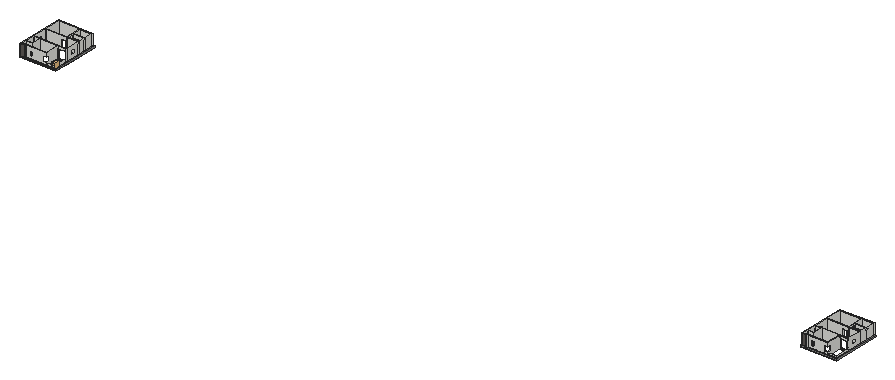
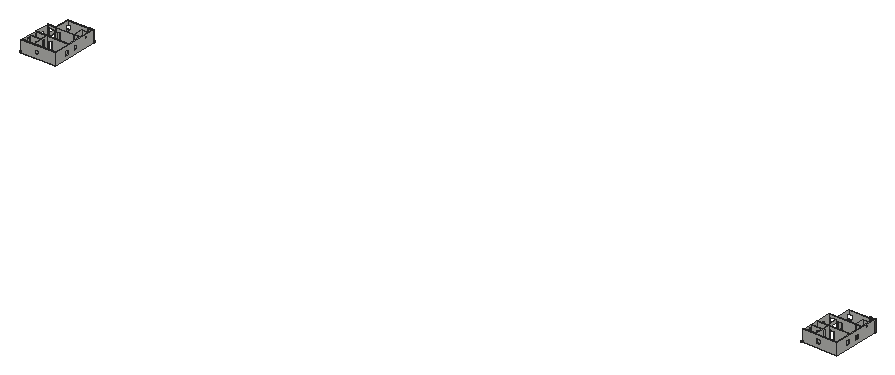
# SketchUp Ruby script. Lengths in inches.
U = 1.inch
M = Sketchup.active_model
def pt(a) = Geom::Point3d.new(a.map { |v| v * U })
def face(e, loops, mat)
  f = e.add_face(loops[0].map { |a| pt(a) })
  loops[1..].each { |l| e.add_face(l.map { |a| pt(a) }).erase! }
  f.material = f.back_material = mat if mat
  f
end
# faces: each face lists its corners as indices into pts; further lists are holes
def faces(e, pts, list, mat = nil) = list.each { |f| face(e, (f[0].is_a?(Array) ? f : [f]).map { |l| l.map { |i| pts[i] } }, mat) }
# xy, xz, yz: faces in a plane at the given z, y or x. An outline is a flat list of corners, or four numbers for a rectangle; further outlines are holes
def ring(l) = l.size == 4 ? [[l[0], l[1]], [l[2], l[1]], [l[2], l[3]], [l[0], l[3]]] : l.each_slice(2).to_a
def flat(e, list, mat, &to3) = list.each { |f| face(e, (f[0].is_a?(Array) ? f : [f]).map { |l| ring(l).map { |u, v| to3.(u, v) } }, mat) }
def xy(e, z, list, mat = nil) = flat(e, list, mat) { |x, y| [x, y, z] }
def xz(e, y, list, mat = nil) = flat(e, list, mat) { |x, z| [x, y, z] }
def yz(e, x, list, mat = nil) = flat(e, list, mat) { |y, z| [x, y, z] }
def lines(e, pts, list) = list.each { |a, b| e.add_line(pt(pts[a]), pt(pts[b])) }
# prism: a flat outline (further loops are holes) pulled along v
def prism(e, loops, v, mat = nil)
  f = face(e, loops, mat); d = Geom::Vector3d.new(v.map { |x| x * U })
  f.pushpull(f.normal.samedirection?(d) ? d.length : -d.length)
end
def box(e, o, s, mat = nil) = prism(e, [[o, [o[0] + s[0], o[1], o[2]], [o[0] + s[0], o[1] + s[1], o[2]], [o[0], o[1] + s[1], o[2]]]], [0, 0, s[2]], mat)
def at(x, y, z, deg = 0) = Geom::Transformation.translation(pt([x, y, z])) * Geom::Transformation.rotation(ORIGIN, Z_AXIS, deg.degrees)
def axes(o, x, y, z) = Geom::Transformation.new([*x, 0, *y, 0, *z, 0, *pt(o).to_a, 1])
def part(name) = M.definitions.add(name)
# library, detail: a bought-in or finely detailed component or shape, given as its bounding box
def library(name, o, s) = part(name).tap { |d| box(d.entities, o, s) }
def detail(e, o, s) = box(e.add_group.entities, o, s)
def put(e, d, t, mat = nil) = e.add_instance(d, t).tap { |i| i.material = mat if mat }
def group(e, t, mat = nil) = e.add_group.tap { |g| g.transformation = t; g.material = mat if mat }.entities
root = M.entities
M.materials.add("Bricks A03 100cm").color = [95, 90, 86]
M.materials.add("Wall Paint Bumpy 01 Gray 100cm").color = [135, 135, 135]
M.materials.add("Wood Amboyan 13.2cm").color = [255, 255, 255]
c1 = part("Vertical board")
xy(c1.entities,0,[[0,0,0.875,8.5625]])
xy(c1.entities,120,[[0,0,0.875,8.5625]])
xz(c1.entities,0,[[0,0,0.875,120]],"Wood Amboyan 13.2cm")
xz(c1.entities,8.5625,[[0,0,0.875,120]])
yz(c1.entities,0,[[0,0,8.5625,120]],"Wood Amboyan 13.2cm")
yz(c1.entities,0.875,[[0,0,8.5625,120]])
c2 = part("Group\#13")
xy(c2.entities,0,[[0,0,45.06,8.5625]])
xy(c2.entities,120.375,[[0,0,45.06,8.5625]])
xz(c2.entities,0,[[0,0,45.06,120.375]],"Bricks A03 100cm")
xz(c2.entities,8.5625,[[0,0,45.06,120.375]])
yz(c2.entities,0,[[0,0,8.5625,120.375]],"Bricks A03 100cm")
yz(c2.entities,45.06,[[0,0,8.5625,120.375]])
c3 = library("Potted Plant 02",[-16.98,-19.78,0],[30.04,38.68,37.52])
xy(root,140.75,[[[420.73,302.125,771.73,779.125],[429.73,311.125,762.73,770.125]],[771.73,302.125,775.4,423.0625],[677.23,311.125,677.23,455.125,672.73,455.125,672.73,459.625,762.73,459.625,762.73,450.625,681.73,450.625,681.73,311.125],[429.73,360.625,452.23,365.125],[485.23,360.625,485.23,365.125,489.73,365.125,489.73,455.125,429.73,455.125,429.73,459.625,633.73,459.625,633.73,455.125,494.23,455.125,494.23,360.625],
  [[8188.44,513.4,8539.44,990.4],[8197.44,522.4,8530.44,981.4]],[8444.94,522.4,8444.94,666.4,8440.44,666.4,8440.44,670.9,8530.44,670.9,8530.44,661.9,8449.44,661.9,8449.44,522.4],[8197.44,571.9,8219.94,576.4],[8252.94,571.9,8252.94,576.4,8257.44,576.4,8257.44,666.4,8197.44,666.4,8197.44,670.9,8401.44,670.9,8401.44,666.4,8261.94,666.4,8261.94,571.9],[429.73,603.625,594.73,608.125],
  [633.73,603.625,633.73,608.125,645.73,608.125,645.73,644.125,650.23,644.125,650.23,608.125,762.73,608.125,762.73,603.625],[645.73,680.125,645.73,770.125,650.23,770.125,650.23,684.625,671.23,684.625,671.23,680.125],[704.23,680.125,762.73,684.625],[8197.44,814.9,8362.44,819.4],[8401.44,814.9,8401.44,819.4,8413.44,819.4,8413.44,855.4,8417.94,855.4,8417.94,819.4,8530.44,819.4,8530.44,814.9],
  [8413.44,891.4,8413.44,981.4,8417.94,981.4,8417.94,895.9,8438.94,895.9,8438.94,891.4],[8471.94,891.4,8530.44,895.9]])
xy(root,140.75,[[420.73,290.125,420.73,293.5625,475.97,293.5625,475.97,302.125,775.4,302.125,775.4,423.0625,786.73,423.0625,786.73,290.125],[771.73,423.0625,786.73,779.125],[8188.44,501.4,8188.44,504.84,8243.6875,504.84,8243.6875,513.4,8539.44,513.4,8539.44,990.4,8554.44,990.4,8554.44,501.4]],"Wall Paint Bumpy 01 Gray 100cm")
xz(root,290.125,[[420.73,140.75,786.73,152.75]],"Wall Paint Bumpy 01 Gray 100cm")
xz(root,293.5625,[[420.73,140.75,475.97,152.75]],"Wall Paint Bumpy 01 Gray 100cm")
xz(root,302.125,[[[420.73,140.75,475.97,140.75,475.97,152.75,681.73,152.75,681.73,176.75,641.23,176.75,641.23,224.75,681.73,224.75,681.73,260.75,420.73,260.75],[512.01,176.75,548.01,224.75]]])
xz(root,302.125,[[475.97,140.75,771.73,152.75]],"Wall Paint Bumpy 01 Gray 100cm")
xz(root,311.125,[[[429.73,140.75,429.73,260.75,677.23,260.75,677.23,224.75,641.23,224.75,641.23,176.75,677.23,176.75,677.23,140.75],[512.01,176.75,548.01,224.75]],[681.73,140.75,762.73,169.375]])
xz(root,360.625,[[429.73,140.75,452.23,140.75,452.23,224.75,485.23,224.75,485.23,140.75,494.23,140.75,494.23,260.75,429.73,260.75]])
xz(root,365.125,[[429.73,140.75,429.73,260.75,489.73,260.75,489.73,140.75,485.23,140.75,485.23,224.75,452.23,224.75,452.23,140.75]])
xz(root,450.625,[[[681.73,140.75,762.73,260.75],[686.23,144.75,758.23,240.75]]])
xz(root,455.125,[[429.73,140.75,489.73,260.75],[494.23,140.75,633.73,140.75,633.73,224.75,672.73,224.75,672.73,140.75,677.23,140.75,677.23,260.75,494.23,260.75]])
xz(root,459.625,[[[429.73,140.75,429.73,260.75,762.73,260.75,762.73,140.75,672.73,140.75,672.73,224.75,633.73,224.75,633.73,140.75],[686.23,144.75,758.23,240.75]]])
xz(root,501.4,[[8188.44,140.75,8554.44,152.75]],"Wall Paint Bumpy 01 Gray 100cm")
xz(root,504.84,[[8188.44,140.75,8243.6875,152.75]],"Wall Paint Bumpy 01 Gray 100cm")
xz(root,513.4,[[[8188.44,140.75,8243.6875,140.75,8243.6875,152.75,8449.44,152.75,8449.44,176.75,8408.94,176.75,8408.94,224.75,8449.44,224.75,8449.44,260.75,8188.44,260.75],[8279.73,176.75,8315.73,224.75]]])
xz(root,513.4,[[8243.6875,140.75,8539.44,152.75]],"Wall Paint Bumpy 01 Gray 100cm")
xz(root,522.4,[[[8197.44,140.75,8197.44,260.75,8444.94,260.75,8444.94,224.75,8408.94,224.75,8408.94,176.75,8444.94,176.75,8444.94,140.75],[8279.73,176.75,8315.73,224.75]],[8449.44,140.75,8530.44,169.375]])
xz(root,571.9,[[8197.44,140.75,8219.94,140.75,8219.94,224.75,8252.94,224.75,8252.94,140.75,8261.94,140.75,8261.94,260.75,8197.44,260.75]])
xz(root,576.4,[[8197.44,140.75,8197.44,260.75,8257.44,260.75,8257.44,140.75,8252.94,140.75,8252.94,224.75,8219.94,224.75,8219.94,140.75]])
xz(root,603.625,[[429.73,140.75,594.73,140.75,594.73,224.75,633.73,224.75,633.73,140.75,762.73,140.75,762.73,260.75,429.73,260.75]])
xz(root,608.125,[[429.73,140.75,429.73,260.75,645.73,260.75,645.73,140.75,633.73,140.75,633.73,224.75,594.73,224.75,594.73,140.75],[650.23,140.75,762.73,260.75]])
xz(root,644.125,[[645.73,140.75,650.23,248.75]])
xz(root,661.9,[[[8449.44,140.75,8530.44,260.75],[8453.94,144.75,8525.94,240.75]]])
xz(root,666.4,[[8197.44,140.75,8257.44,260.75],[8261.94,140.75,8401.44,140.75,8401.44,224.75,8440.44,224.75,8440.44,140.75,8444.94,140.75,8444.94,260.75,8261.94,260.75]])
xz(root,670.9,[[[8197.44,140.75,8197.44,260.75,8530.44,260.75,8530.44,140.75,8440.44,140.75,8440.44,224.75,8401.44,224.75,8401.44,140.75],[8453.94,144.75,8525.94,240.75]]])
xz(root,680.125,[[645.73,140.75,650.23,248.75],[650.23,140.75,671.23,140.75,671.23,224.75,704.23,224.75,704.23,140.75,762.73,140.75,762.73,260.75,650.23,260.75]])
xz(root,684.625,[[650.23,140.75,650.23,260.75,762.73,260.75,762.73,140.75,704.23,140.75,704.23,224.75,671.23,224.75,671.23,140.75]])
xz(root,770.125,[[[429.73,140.75,645.73,260.75],[590.04,176.75,638.04,224.75]],[645.73,140.75,650.23,260.75],[650.23,140.75,762.73,260.75]])
xz(root,779.125,[[[420.73,140.75,771.73,260.75],[590.04,176.75,638.04,224.75]]])
xz(root,779.125,[[771.73,140.75,786.73,152.75]],"Wall Paint Bumpy 01 Gray 100cm")
xz(root,814.9,[[8197.44,140.75,8362.44,140.75,8362.44,224.75,8401.44,224.75,8401.44,140.75,8530.44,140.75,8530.44,260.75,8197.44,260.75]])
xz(root,819.4,[[8197.44,140.75,8197.44,260.75,8413.44,260.75,8413.44,140.75,8401.44,140.75,8401.44,224.75,8362.44,224.75,8362.44,140.75],[8417.94,140.75,8530.44,260.75]])
xz(root,855.4,[[8413.44,140.75,8417.94,248.75]])
xz(root,891.4,[[8413.44,140.75,8417.94,248.75],[8417.94,140.75,8438.94,140.75,8438.94,224.75,8471.94,224.75,8471.94,140.75,8530.44,140.75,8530.44,260.75,8417.94,260.75]])
xz(root,895.9,[[8417.94,140.75,8417.94,260.75,8530.44,260.75,8530.44,140.75,8471.94,140.75,8471.94,224.75,8438.94,224.75,8438.94,140.75]])
xz(root,981.4,[[[8197.44,140.75,8413.44,260.75],[8357.75,176.75,8405.75,224.75]],[8413.44,140.75,8417.94,260.75],[8417.94,140.75,8530.44,260.75]])
xz(root,990.4,[[[8188.44,140.75,8539.44,260.75],[8357.75,176.75,8405.75,224.75]]])
xz(root,990.4,[[8539.44,140.75,8554.44,152.75]],"Wall Paint Bumpy 01 Gray 100cm")
yz(root,420.73,[[[302.125,140.75,779.125,260.75],[618.96,176.75,666.96,224.75],[507.625,176.75,555.625,224.75],[387.69,230.75,411.65,248.75]]])
yz(root,420.73,[[290.125,140.75,293.5625,152.75]],"Wall Paint Bumpy 01 Gray 100cm")
yz(root,429.73,[[311.125,140.75,360.625,260.75],[360.625,140.75,365.125,260.75],[[365.125,140.75,455.125,260.75],[387.69,230.75,411.65,248.75]],[455.125,140.75,459.625,260.75],[[459.625,140.75,603.625,260.75],[507.625,176.75,555.625,224.75]],
  [603.625,140.75,608.125,260.75],[[608.125,140.75,770.125,260.75],[618.96,176.75,666.96,224.75]]])
yz(root,452.23,[[360.625,140.75,365.125,224.75]])
yz(root,475.97,[[293.5625,140.75,302.125,152.75]],"Wall Paint Bumpy 01 Gray 100cm")
yz(root,485.23,[[360.625,140.75,365.125,224.75]])
yz(root,489.73,[[365.125,140.75,455.125,260.75]])
yz(root,494.23,[[360.625,140.75,455.125,260.75]])
yz(root,594.73,[[603.625,140.75,608.125,224.75]])
yz(root,633.73,[[455.125,140.75,459.625,224.75],[603.625,140.75,608.125,224.75]])
yz(root,645.73,[[608.125,140.75,608.125,260.75,770.125,260.75,770.125,140.75,680.125,140.75,680.125,248.75,644.125,248.75,644.125,140.75]])
yz(root,650.23,[[608.125,140.75,644.125,140.75,644.125,248.75,680.125,248.75,680.125,260.75,608.125,260.75],[684.625,140.75,770.125,260.75]])
yz(root,671.23,[[680.125,140.75,684.625,224.75]])
yz(root,672.73,[[455.125,140.75,459.625,224.75]])
yz(root,677.23,[[311.125,140.75,311.125,176.75,335.125,176.75,335.125,224.75,311.125,224.75,311.125,260.75,455.125,260.75,455.125,140.75]])
yz(root,681.73,[[311.125,140.75,450.25,140.75,450.25,259.75,325.25,259.75,325.25,260.75,302.125,260.75,302.125,224.75,335.125,224.75,335.125,176.75,302.125,176.75,302.125,170.375,311.125,170.375],[450.25,140.75,450.625,260.75]])
yz(root,704.23,[[680.125,140.75,684.625,224.75]])
yz(root,762.73,[[311.125,140.75,450.625,169.375],[450.625,140.75,459.625,260.75],[[459.625,140.75,603.625,260.75],[507.625,176.75,555.625,224.75]],[603.625,140.75,608.125,260.75],[608.125,140.75,680.125,260.75],
  [680.125,140.75,684.625,260.75],[[684.625,140.75,770.125,260.75],[691.19,230.75,715.15,248.75]]])
yz(root,771.73,[[302.125,140.75,779.125,152.75]],"Wall Paint Bumpy 01 Gray 100cm")
yz(root,786.73,[[290.125,140.75,779.125,152.75]],"Wall Paint Bumpy 01 Gray 100cm")
yz(root,8188.44,[[[513.4,140.75,990.4,260.75],[830.24,176.75,878.24,224.75],[718.9,176.75,766.9,224.75],[598.97,230.75,622.93,248.75]]])
yz(root,8188.44,[[501.4,140.75,504.84,152.75]],"Wall Paint Bumpy 01 Gray 100cm")
yz(root,8197.44,[[522.4,140.75,571.9,260.75],[571.9,140.75,576.4,260.75],[[576.4,140.75,666.4,260.75],[598.97,230.75,622.93,248.75]],[666.4,140.75,670.9,260.75],[[670.9,140.75,814.9,260.75],[718.9,176.75,766.9,224.75]],
  [814.9,140.75,819.4,260.75],[[819.4,140.75,981.4,260.75],[830.24,176.75,878.24,224.75]]])
yz(root,8219.94,[[571.9,140.75,576.4,224.75]])
yz(root,8243.6875,[[504.84,140.75,513.4,152.75]],"Wall Paint Bumpy 01 Gray 100cm")
yz(root,8252.94,[[571.9,140.75,576.4,224.75]])
yz(root,8257.44,[[576.4,140.75,666.4,260.75]])
yz(root,8261.94,[[571.9,140.75,666.4,260.75]])
yz(root,8362.44,[[814.9,140.75,819.4,224.75]])
yz(root,8401.44,[[666.4,140.75,670.9,224.75],[814.9,140.75,819.4,224.75]])
yz(root,8413.44,[[819.4,140.75,819.4,260.75,981.4,260.75,981.4,140.75,891.4,140.75,891.4,248.75,855.4,248.75,855.4,140.75]])
yz(root,8417.94,[[819.4,140.75,855.4,140.75,855.4,248.75,891.4,248.75,891.4,260.75,819.4,260.75],[895.9,140.75,981.4,260.75]])
yz(root,8438.94,[[891.4,140.75,895.9,224.75]])
yz(root,8440.44,[[666.4,140.75,670.9,224.75]])
yz(root,8444.94,[[522.4,140.75,522.4,176.75,546.4,176.75,546.4,224.75,522.4,224.75,522.4,260.75,666.4,260.75,666.4,140.75]])
yz(root,8449.44,[[522.4,140.75,661.53,140.75,661.53,260.75,513.4,260.75,513.4,224.75,546.4,224.75,546.4,176.75,513.4,176.75,513.4,170.375,522.4,170.375],[661.53,140.75,661.9,260.75]])
yz(root,8471.94,[[891.4,140.75,895.9,224.75]])
yz(root,8530.44,[[522.4,140.75,661.9,169.375],[661.9,140.75,670.9,260.75],[[670.9,140.75,814.9,260.75],[718.9,176.75,766.9,224.75]],[814.9,140.75,819.4,260.75],[819.4,140.75,891.4,260.75],
  [891.4,140.75,895.9,260.75],[[895.9,140.75,981.4,260.75],[902.47,230.75,926.43,248.75]]])
yz(root,8539.44,[[513.4,140.75,990.4,152.75]],"Wall Paint Bumpy 01 Gray 100cm")
yz(root,8554.44,[[501.4,140.75,990.4,152.75]],"Wall Paint Bumpy 01 Gray 100cm")
put(root,c1,at(471.9,293.5625,140.75))
put(root,c1,at(467.1,293.5625,140.75))
put(root,c1,at(475.1,293.5625,140.75))
put(root,c1,at(473.5,293.5625,140.75))
put(root,c1,at(470.3,293.5625,140.75))
put(root,c1,at(468.7,293.5625,140.75))
put(root,c2,at(420.73,293.5625,140.75))
put(root,c1,at(8234.8125,504.84,140.75))
put(root,c1,at(8236.41,504.84,140.75))
put(root,c1,at(8238.01,504.84,140.75))
put(root,c1,at(8239.61,504.84,140.75))
put(root,c1,at(8241.21,504.84,140.75))
put(root,c1,at(8242.8125,504.84,140.75))
put(root,c2,at(8188.44,504.84,140.75))
put(root,c3,axes([746.27,336.95,140.75],[1.29,0,0],[0,1.29,0],[0,0,1.29]))
